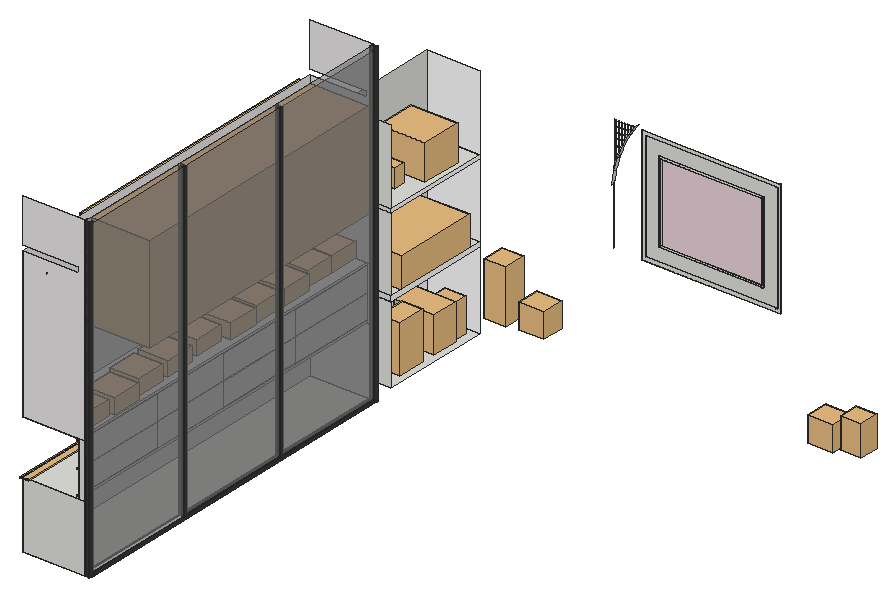
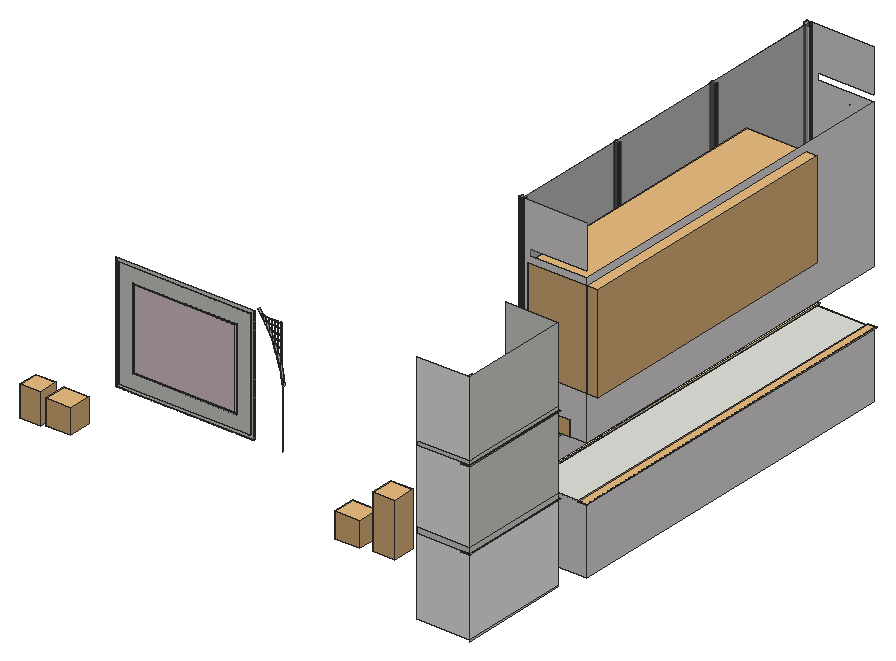
# SketchUp Ruby script. Lengths in inches.
U = 1.inch
M = Sketchup.active_model
def pt(a) = Geom::Point3d.new(a.map { |v| v * U })
def face(e, loops, mat)
  f = e.add_face(loops[0].map { |a| pt(a) })
  loops[1..].each { |l| e.add_face(l.map { |a| pt(a) }).erase! }
  f.material = f.back_material = mat if mat
  f
end
# faces: each face lists its corners as indices into pts; further lists are holes
def faces(e, pts, list, mat = nil) = list.each { |f| face(e, (f[0].is_a?(Array) ? f : [f]).map { |l| l.map { |i| pts[i] } }, mat) }
# xy, xz, yz: faces in a plane at the given z, y or x. An outline is a flat list of corners, or four numbers for a rectangle; further outlines are holes
def ring(l) = l.size == 4 ? [[l[0], l[1]], [l[2], l[1]], [l[2], l[3]], [l[0], l[3]]] : l.each_slice(2).to_a
def flat(e, list, mat, &to3) = list.each { |f| face(e, (f[0].is_a?(Array) ? f : [f]).map { |l| ring(l).map { |u, v| to3.(u, v) } }, mat) }
def xy(e, z, list, mat = nil) = flat(e, list, mat) { |x, y| [x, y, z] }
def xz(e, y, list, mat = nil) = flat(e, list, mat) { |x, z| [x, y, z] }
def yz(e, x, list, mat = nil) = flat(e, list, mat) { |y, z| [x, y, z] }
def lines(e, pts, list) = list.each { |a, b| e.add_line(pt(pts[a]), pt(pts[b])) }
# prism: a flat outline (further loops are holes) pulled along v
def prism(e, loops, v, mat = nil)
  f = face(e, loops, mat); d = Geom::Vector3d.new(v.map { |x| x * U })
  f.pushpull(f.normal.samedirection?(d) ? d.length : -d.length)
end
def box(e, o, s, mat = nil) = prism(e, [[o, [o[0] + s[0], o[1], o[2]], [o[0] + s[0], o[1] + s[1], o[2]], [o[0], o[1] + s[1], o[2]]]], [0, 0, s[2]], mat)
def at(x, y, z, deg = 0) = Geom::Transformation.translation(pt([x, y, z])) * Geom::Transformation.rotation(ORIGIN, Z_AXIS, deg.degrees)
def axes(o, x, y, z) = Geom::Transformation.new([*x, 0, *y, 0, *z, 0, *pt(o).to_a, 1])
def part(name) = M.definitions.add(name)
# library, detail: a bought-in or finely detailed component or shape, given as its bounding box
def library(name, o, s) = part(name).tap { |d| box(d.entities, o, s) }
def detail(e, o, s) = box(e.add_group.entities, o, s)
def put(e, d, t, mat = nil) = e.add_instance(d, t).tap { |i| i.material = mat if mat }
def group(e, t, mat = nil) = e.add_group.tap { |g| g.transformation = t; g.material = mat if mat }.entities
root = M.entities
M.materials.add("Generic").color = [234, 232, 232]
M.materials.add("Gold 10k").color = [251, 232, 180]
M.materials.add("[Color M00]").color = [255, 255, 255]
M.materials.add("[Color M02]").color = [237, 213, 220]
M.materials.add("[Color M07]").color = [58, 58, 58]
M.materials.add("[Translucent Glass Gray]").color = [128, 128, 128]
M.materials["[Translucent Glass Gray]"].alpha = 0.5
c1 = library("Interior Props 221 031",[-3.74,-3.52,-0.04],[7.48,7.03,11.78])
c2 = library("Interior Props 221 030",[-2.57,-3.63,-0.04],[5.13,7.27,11.89])
c3 = library("Interior Props 221 029",[-1.46,-2.15,0],[2.92,4.3,3.83])
c4 = library("Lamp Table 025",[-4.92,-4.92,-0.03],[22.02,19.61,21.68])
c5 = library("Potted Succulent 003",[-4.09,-3.62,0],[7.1,6.83,10.79])
c6 = library("Potted Basil 50-07",[-3.85,-3.53,0.03],[7.56,8,18.65])
c7 = library("Group\#7",[-0.5,-0.5,-0.1],[3,127.16,0.2])
c8 = library("Group\#1",[-0.5,-0.5,-0.1],[3,40,0.2])
c9 = library("Bowls and Vases 20-14",[-14.94,-8.87,0],[29.88,17.74,10.58])
c10 = library("Clothes 159 005",[-5.11,-5.34,0.03],[10.26,10.67,5.26])
c11 = library("Group\#4",[-0.5,-0.5,-0.1],[3,40,0.2])
c12 = library("Interior Props 160 011",[-3.43,-7.07,0],[14.06,16.26,12.45])
c13 = library("Perfume 101 004",[-2,-2,-0.02],[4,4,6.5])
c14 = library("Clothing 209 002",[69.11,63.18,62.21],[24.57,96.36,33.87])
xy(root,4.07,[[11.1875,11.43,33,137.59],[33,11.43,33.4375,12.43],[33.4375,11.43,34.4375,12.43],[34.4375,11.43,34.8125,12.43],[33,136.59,33.4375,137.59],
  [33.4375,136.59,34.4375,137.59],[34.4375,136.59,34.8125,137.59]])
xy(root,4.07,[[33,12.43,33.4375,136.59],[33.4375,12.43,34.4375,136.59],[34.4375,12.43,34.8125,136.59]],"[Color M07]")
xy(root,4.17,[[14.5,145.84,33,184.83]])
xy(root,5.07,[[33,12.43,34.4375,52.82],[33,52.82,34.4375,53.82],[34.4375,52.82,34.8125,53.82],[33,95.21,34.4375,96.21],[34.4375,95.21,34.8125,96.21]])
xy(root,5.07,[[34.4375,12.43,34.8125,52.82],[33,53.82,34.4375,95.21],[34.4375,53.82,34.8125,95.21],[33,96.21,34.4375,136.59],[34.4375,96.21,34.8125,136.59]],"[Color M07]")
xy(root,27.47,[[13.1875,11.43,31,137.59]])
xy(root,28.22,[[30.25,11.43,31,137.59]],"Gold 10k")
xy(root,28.62,[[30.25,11.43,31,45.36],[30.25,45.76,31,74.51],[30.25,74.91,31,106.25],[30.25,106.65,31,137.59]],"Gold 10k")
xy(root,31.38,[[16.5,145.84,33,184.83]])
xy(root,33.15,[[14.5,145.84,33,184.83]])
xy(root,36.62,[[30.25,11.43,31,45.36],[30.25,45.76,31,74.51],[30.25,74.91,31,106.25],[30.25,106.65,31,137.59]],"Gold 10k")
xy(root,37.02,[[30.25,11.43,31,45.36],[30.25,45.76,31,74.51],[30.25,74.91,31,106.25],[30.25,106.65,31,137.59]],"Gold 10k")
xy(root,44.04,[[86.13,189.625,86.13,189.8125,86.26,189.8125,86.26,189.875,86.82,189.875,86.82,189.8125,87.42,189.8125,87.42,189.875,87.99,189.875,87.99,189.8125,88.58,189.8125,88.58,189.875,89.15,189.875,89.15,189.8125,89.75,189.8125,89.75,189.875,90.3125,189.875,90.3125,189.8125,90.91,189.8125,90.91,189.875,91.48,189.875,91.48,189.8125,92.08,189.8125,92.08,189.875,92.64,189.875,92.64,189.8125,93.24,189.8125,93.24,189.875,93.8,189.875,93.8,189.8125,94.4,189.8125,94.4,189.875,94.97,189.875,94.97,189.8125,95.57,189.8125,95.57,189.875,96.13,189.875,96.13,189.8125,96.73,189.8125,96.73,189.875,97.29,189.875,97.29,189.8125,97.89,189.8125,97.89,189.875,98.46,189.875,98.46,189.8125,99.06,189.8125,99.06,189.875,99.62,189.875,99.62,189.8125,100.22,189.8125,100.22,189.875,100.79,189.875,100.79,189.8125,101.38,189.8125,101.38,189.875,101.95,189.875,101.95,189.8125,102.55,189.8125,102.55,189.875,103.11,189.875,103.11,189.8125,103.71,189.8125,103.71,189.875,104.28,189.875,104.28,189.8125,104.875,189.8125,104.875,189.875,105.28,189.875,105.28,189.8125,105.875,189.8125,105.875,189.875,106.28,189.875,106.28,189.8125,106.875,189.8125,106.875,189.875,107.28,189.875,107.28,189.8125,107.875,189.8125,107.875,189.875,108.28,189.875,108.28,189.8125,108.875,189.8125,108.875,189.875,109.28,189.875,109.28,189.8125,109.875,189.8125,109.875,189.875,110.28,189.875,110.28,189.8125,110.875,189.8125,110.875,189.875,111.28,189.875,111.28,189.8125,111.875,189.8125,111.875,189.875,112.28,189.875,112.28,189.8125,112.875,189.8125,112.875,189.875,113.28,189.875,113.28,189.8125,113.875,189.8125,113.875,189.875,114.28,189.875,114.28,189.8125,114.875,189.8125,114.875,189.875,115.28,189.875,115.28,189.8125,115.875,189.8125,115.875,189.875,116.28,189.875,116.28,189.8125,116.875,189.8125,116.875,189.875,117.28,189.875,117.28,189.8125,117.875,189.8125,117.875,189.875,118.28,189.875,118.28,189.8125,118.875,189.8125,118.875,189.875,119.28,189.875,119.28,189.8125,119.875,189.8125,119.875,189.875,120.28,189.875,120.28,189.8125,120.875,189.8125,120.875,189.875,121.28,189.875,121.28,189.8125,121.875,189.8125,121.875,189.875,122.28,189.875,122.28,189.8125,122.875,189.8125,122.875,189.875,123.28,189.875,123.28,189.8125,123.875,189.8125,123.875,189.875,124.28,189.875,124.28,189.75,124.875,189.75,124.875,189.875,125.28,189.875,125.28,189.75,125.875,189.75,125.875,189.875,126.28,189.875,126.28,189.75,126.875,189.75,126.875,189.875,127.28,189.875,127.28,189.75,127.875,189.75,127.875,189.875,128.28,189.875,128.28,189.75,128.875,189.75,128.875,189.875,129.28,189.875,129.28,189.75,129.875,189.75,129.875,189.875,130.28,189.875,130.28,189.75,130.875,189.75,130.875,189.875,131.28,189.875,131.28,189.75,131.875,189.75,131.875,189.875,132.28,189.875,132.28,189.75,132.875,189.75,132.875,189.875,133.28,189.875,133.28,189.75,133.875,189.75,133.875,189.875,134.28,189.875,134.28,189.625],[134.28,189.625,134.75,189.875],[131.28,189.75,131.75,189.875],[131.75,189.75,131.875,189.875],[132.28,189.75,132.75,189.875],
  [132.75,189.75,132.875,189.875],[133.28,189.75,133.75,189.875],[133.75,189.75,133.875,189.875],[86.13,189.8125,86.14,189.875],[86.14,189.8125,86.26,189.875]])
xy(root,45.1875,[[87.28,189.625,133.61,189.875]])
xy(root,45.36,[[30.25,106.65,31,137.59]],"Gold 10k")
xy(root,45.42,[[30.25,45.76,31,45.77]])
xy(root,45.42,[[30.25,11.43,31,45.36],[30.25,45.77,31,74.51],[30.25,74.91,31,106.25]],"Gold 10k")
xy(root,45.82,[[30.25,11.43,31,137.59]],"Gold 10k")
xy(root,46.57,[[11.1875,11.43,31,137.59]],"Generic")
xy(root,50.04,[[92.125,189.625,128.76,189.875]])
xy(root,50.62,[[92.71,189.625,128.18,189.875]])
xy(root,59.13,[[16.5,145.84,33,184.83]])
xy(root,60.4,[[14.5,145.84,33,184.83]])
xy(root,78.09,[[92.71,189.625,128.18,189.875]])
xy(root,78.67,[[92.125,189.625,128.76,189.875]])
xy(root,83.52,[[87.28,189.625,133.61,189.875]])
xz(root,11.43,[[11.1875,4.07,33,27.47],[31,27.47,31,28.22,30.25,28.22,30.25,28.62,31,28.62,31,36.62,30.25,36.62,30.25,37.02,31,37.02,31,45.42,30.25,45.42,30.25,45.82,31,45.82,31,46.57,33,46.57,33,27.47]])
xz(root,11.43,[[[11.1875,46.57,11.1875,98.59,31,98.59,31,100.64,11.1875,100.64,11.1875,115.93,33,115.93,33,46.57],[19.57,94.12,19.68,94.13,19.77,94.17,19.86,94.23,19.92,94.32,19.96,94.41,19.97,94.52,19.96,94.62,19.92,94.72,19.86,94.8,19.77,94.86,19.68,94.9,19.57,94.92,19.47,94.9,19.37,94.86,19.29,94.8,19.23,94.72,19.1875,94.62,19.17,94.52,19.1875,94.41,19.23,94.32,19.29,94.23,19.37,94.17,19.47,94.13]]],"Generic")
xz(root,11.43,[[33,4.07,33.4375,115.93],[33.4375,4.07,34.4375,115.93],[34.4375,4.07,34.8125,115.93]],"[Color M07]")
xz(root,12.43,[[33,4.07,34.4375,5.07],[34.4375,4.07,34.8125,5.07],[33,5.07,34.4375,114.93]])
xz(root,12.43,[[34.4375,5.07,34.8125,114.93]],"[Color M07]")
xz(root,45.36,[[30.25,28.62,31,36.62],[30.25,37.02,31,45.42]],"Gold 10k")
xz(root,45.76,[[30.25,28.62,31,36.62],[30.25,37.02,31,45.42]],"Gold 10k")
xz(root,52.82,[[33,5.07,34.4375,114.93],[34.4375,5.07,34.8125,114.93]],"[Color M07]")
xz(root,53.82,[[33,5.07,34.4375,114.93],[34.4375,5.07,34.8125,114.93]],"[Color M07]")
xz(root,74.51,[[30.25,28.62,31,36.62],[30.25,37.02,31,45.42]],"Gold 10k")
xz(root,74.91,[[30.25,28.62,31,36.62],[30.25,37.02,31,45.42]],"Gold 10k")
xz(root,95.21,[[33,5.07,34.4375,114.93],[34.4375,5.07,34.8125,114.93]],"[Color M07]")
xz(root,96.21,[[33,5.07,34.4375,114.93],[34.4375,5.07,34.8125,114.93]],"[Color M07]")
xz(root,106.25,[[30.25,28.62,31,36.62],[30.25,37.02,31,45.42]],"Gold 10k")
xz(root,106.65,[[30.25,28.62,31,36.62],[30.25,37.02,31,45.36]],"Gold 10k")
xz(root,136.59,[[33,4.07,34.4375,5.07],[34.4375,4.07,34.8125,5.07]])
xz(root,136.59,[[33,5.07,34.4375,114.93],[34.4375,5.07,34.8125,114.93]],"[Color M07]")
xz(root,137.59,[[11.1875,4.07,33,27.47],[31,27.47,33,27.47,33,46.57,31,46.57,31,45.82,30.25,45.82,30.25,45.36,31,45.36,31,37.02,30.25,37.02,30.25,36.62,31,36.62,31,28.62,30.25,28.62,30.25,28.22,31,28.22],[[11.1875,46.57,33,46.57,33,115.93,11.1875,115.93,11.1875,100.64,31,100.64,31,98.59,11.1875,98.59],[19.57,94.12,19.47,94.13,19.37,94.17,19.29,94.23,19.23,94.32,19.1875,94.41,19.17,94.52,19.1875,94.62,19.23,94.72,19.29,94.8,19.37,94.86,19.47,94.9,19.57,94.92,19.68,94.9,19.77,94.86,19.86,94.8,19.92,94.72,19.96,94.62,19.97,94.52,19.96,94.41,19.92,94.32,19.86,94.23,19.77,94.17,19.68,94.13]]],"Generic")
xz(root,137.59,[[33,4.07,33.4375,115.93],[33.4375,4.07,34.4375,115.93],[34.4375,4.07,34.8125,115.93]],"[Color M07]")
xz(root,145.84,[[14.5,4.17,33,31.38],[14.5,31.38,33,33.15],[14.5,33.15,33,59.13],[14.5,59.13,33,60.4],[14.5,60.4,33,86.88]])
xz(root,184.83,[[14.5,31.38,33,33.15],[14.5,59.13,33,60.4]])
xz(root,184.83,[[14.5,4.17,33,31.38],[14.5,33.15,33,59.13],[14.5,60.4,33,86.88]],"[Color M00]")
xz(root,189.625,[[[86.13,44.04,134.75,84.67],[87.28,45.1875,133.61,83.52]],[[92.125,50.04,128.76,78.67],[92.71,50.62,128.18,78.09]]])
xz(root,189.875,[[76,44.04,76.0625,44.04,76.0625,64.2,76.6,67.64,76.6,71.82,76,69.625],[86.13,44.04,86.26,84.67],[134.28,44.04,134.75,84.67],[[87.28,45.1875,133.61,83.52],[92.125,50.04,128.76,78.67]],[77,69.625,77.6,71.82,77.6,74.82,77.03,73.375,77,73.29],
  [78,73.29,78.03,73.375,78.6,74.82,78.6,77.35,78,75.84],[79,75.84,79.6,77.35,79.6,79.33,79,78.2],[80,78.2,80.6,79.33,80.6,81.21,80,80.08],[81,80.08,81.6,81.21,81.6,83.06,81,82.1875],[82.17,82.1875,82.77,83.06,82.77,84.67,82.7,84.67,82.17,83.89],
  [83.33,83.89,83.86,84.67,83.33,84.67]])
xz(root,189.875,[[92.71,50.62,128.18,78.09]],"[Color M02]")
yz(root,11.1875,[[11.43,4.07,137.59,27.47],[11.43,46.57,137.59,98.59]],"Generic")
yz(root,14.5,[[145.84,3.63,184.83,4.17],[145.84,31.38,184.83,33.15],[145.84,33.15,184.83,59.13],[145.84,59.13,184.83,60.4],[145.84,60.4,184.83,86.88]])
yz(root,14.5,[[145.84,4.17,184.83,31.38]],"[Color M00]")
yz(root,30.25,[[[11.43,28.22,137.59,28.22,137.59,28.62,106.65,28.62,106.65,36.62,137.59,36.62,137.59,37.02,106.65,37.02,106.65,45.36,137.59,45.36,137.59,45.82,11.43,45.82,11.43,45.42,45.36,45.42,45.36,37.02,11.43,37.02,11.43,36.62,45.36,36.62,45.36,28.62,11.43,28.62],[74.91,37.02,106.25,45.42],[74.91,28.62,106.25,36.62],[45.76,37.02,74.51,45.42],[45.76,28.62,74.51,36.62]]],"Gold 10k")
yz(root,31,[[11.43,27.47,137.59,28.22],[11.43,28.62,45.36,36.62],[45.76,28.62,74.51,36.62],[74.91,28.62,106.25,36.62],[106.65,28.62,137.59,36.62],
  [11.43,37.02,45.36,45.42],[45.76,37.02,74.51,45.42],[74.91,37.02,106.25,45.42],[106.65,37.02,137.59,45.36],[11.43,45.82,137.59,46.57]],"Generic")
yz(root,33,[[145.84,31.38,184.83,33.15],[145.84,59.13,184.83,60.4]],"[Color M00]")
yz(root,33,[[11.43,4.07,12.43,115.93],[12.43,4.07,136.59,5.07],[136.59,4.07,137.59,115.93],[52.82,5.07,53.82,114.93],[95.21,5.07,96.21,114.93]],"[Color M07]")
yz(root,33.4375,[[11.43,4.07,137.59,115.93]],"[Translucent Glass Gray]")
yz(root,34.4375,[[11.43,4.07,12.43,115.93],[12.43,4.07,136.59,5.07],[136.59,4.07,137.59,115.93],[52.82,5.07,53.82,114.93],[95.21,5.07,96.21,114.93]])
yz(root,34.4375,[[12.43,5.07,52.82,114.93],[53.82,5.07,95.21,114.93],[96.21,5.07,136.59,114.93]],"[Translucent Glass Gray]")
yz(root,34.8125,[[11.43,4.07,12.43,115.93],[12.43,4.07,136.59,5.07],[136.59,4.07,137.59,115.93],[52.82,5.07,53.82,114.93],[95.21,5.07,96.21,114.93]],"[Color M07]")
yz(root,76.0625,[[189.8125,44.04,189.875,64.2]])
yz(root,86.13,[[189.625,44.04,189.8125,84.67],[189.8125,44.04,189.875,84.67]])
yz(root,87.28,[[189.625,45.1875,189.875,83.52]])
yz(root,92.125,[[189.625,50.04,189.875,78.67]])
yz(root,92.71,[[189.625,50.62,189.875,78.09]])
yz(root,128.18,[[189.625,50.62,189.875,78.09]])
yz(root,128.76,[[189.625,50.04,189.875,78.67]])
yz(root,133.61,[[189.625,45.1875,189.875,83.52]])
yz(root,134.75,[[189.625,44.04,189.875,84.67]])
p = [[76.79,189,68.84],[76.0625,189,64.2],[76.0625,189.8125,64.2],[76.6,189.8125,67.64],[76.6,189.875,67.64],[76.79,189.875,68.84],
  [76.0625,189.875,64.2],[78.03,189,73.375],[77,189.875,69.625],[77,189.8125,69.625],[77.6,189.8125,71.82],[77.6,189.875,71.82],
  [78,189.875,73.29],[78,189.8125,73.29],[78.03,189.8125,73.375],[78.03,189.875,73.375],[79.76,189,77.74],[78.6,189.8125,74.82],
  [78.6,189.875,74.82],[79,189.875,75.84],[79,189.8125,75.84],[79.6,189.8125,77.35],[79.6,189.875,77.35],[79.76,189.875,77.74],
  [81.96,189,81.89],[80,189.875,78.2],[80,189.8125,78.2],[80.6,189.8125,79.33],[80.6,189.875,79.33],[81,189.875,80.08],
  [81,189.8125,80.08],[81.6,189.8125,81.21],[81.6,189.875,81.21],[81.96,189.875,81.89],[84.62,189,85.77],[82.17,189.875,82.1875],
  [82.17,189.8125,82.1875],[82.77,189.8125,83.06],[82.77,189.875,83.06],[83.33,189.875,83.89],[83.33,189.8125,83.89],[83.86,189.8125,84.67],
  [83.86,189.875,84.67],[84.28,189.875,85.28],[84.28,189.8125,85.28],[84.62,189.8125,85.77],[31,74.51,45.42],[31,74.53,45.42],
  [82.17,189.875,83.89],[82.17,189.875,84.67],[81.6,189.875,84.67],[81.6,189.875,83.06],[81,189.875,83.89],[81,189.875,84.67],
  [81.53,189.875,84.67],[81,189.875,82.1875],[80.53,189.875,84.67],[80,189.875,83.89],[80,189.875,82.1875],[80.6,189.875,83.06],
  [80.6,189.875,81.21],[80,189.875,80.08],[80.6,189.875,84.67],[80,189.875,84.67],[79,189.875,83.89],[79,189.875,84.67],
  [79.6,189.875,81.21],[79.6,189.875,79.33],[79.6,189.875,84.67],[79.6,189.875,83.06],[79.53,189.875,84.67],[79,189.875,82.1875],
  [79,189.875,78.2],[79,189.875,80.08],[78.6,189.875,84.67],[78.6,189.875,83.06],[78,189.875,83.89],[78,189.875,84.67],
  [78.6,189.875,81.21],[78.6,189.875,79.33],[78.53,189.875,84.67],[78,189.875,82.1875],[78,189.875,80.08],[78,189.875,78.2],
  [78,189.875,75.84],[78.6,189.875,77.35],[77.53,189.875,84.67],[77,189.875,83.89],[77,189.875,80.08],[77,189.875,82.1875],
  [77.6,189.875,77.35],[77,189.875,75.84],[77,189.875,84.67],[77,189.875,73.29],[77.6,189.875,81.21],[77.6,189.875,79.33],
  [77.6,189.875,84.67],[77.6,189.875,83.06],[77,189.875,78.2],[77.6,189.875,74.82],[76.6,189.875,79.33],[76.6,189.875,77.35],
  [76.6,189.875,74.82],[76,189.875,75.84],[76,189.875,78.2],[76.6,189.875,83.06],[76.6,189.875,81.21],[76.03,189.875,73.375],
  [76,189.875,73.29],[76.6,189.875,71.82],[76,189.875,80.08],[76.53,189.875,84.67],[76,189.875,83.89],[76.6,189.875,84.67],
  [76,189.875,82.1875],[76,189.875,84.67],[76,189.875,69.625]]
faces(root,p,[[0,1,2,3,4,5],[6,4,3,2],[7,0,5,8,9,10,11,12,13,14],[8,11,10,9],[12,15,14,13],[16,7,14,17,18,19,20,21,22,23],[15,18,17,14],[19,22,21,20],
  [24,16,23,25,26,27,28,29,30,31,32,33],[25,28,27,26],[29,32,31,30],[34,24,33,35,36,37,38,39,40,41,42,43,44,45],[35,38,37,36],[39,42,41,40]])
lines(root,p,[[46,47],[48,49],[50,51],[52,53],[54,52],[55,52],[56,57],[58,57],[59,58],[59,60],[61,58],[62,59],
  [57,63],[64,65],[66,67],[68,69],[70,64],[71,64],[69,71],[72,73],[69,66],[73,71],[66,73],[74,75],
  [76,77],[78,79],[80,76],[81,76],[82,81],[75,81],[79,83],[84,83],[75,78],[79,85],[78,82],[83,82],
  [86,87],[88,89],[90,91],[89,87],[87,92],[93,91],[94,95],[96,97],[97,89],[95,98],[91,98],[95,90],
  [94,88],[98,88],[90,99],[97,94],[100,101],[101,102],[103,104],[105,106],[102,107],[107,108],[102,109],[104,110],
  [106,110],[111,112],[113,105],[105,114],[114,112],[108,103],[110,114],[101,103],[112,115],[106,100],[100,104],[116,108]])
put(root,c1,at(26.23,179,4.17))
put(root,c2,axes([26.91,157.73,4.18],[1.39,0,0],[0,1.39,0],[0,0,1.39]))
put(root,c3,axes([23.53,172.35,4.16],[0,3.29,0],[-3.29,0,0],[0,0,3.29]))
put(root,c4,axes([56.93,176.47,17.7],[0.4,0,0],[0,0.4,0],[0,0,0.4]))
put(root,c4,axes([158.24,176.47,17.7],[0.4,0,0],[0,0.4,0],[0,0,0.4]))
put(root,c5,at(170.09,180.48,17.72))
put(root,c6,at(47.38,176.97,17.6875))
put(root,c7,at(11.1875,11.43,27.47))
put(root,c8,at(14.5,145.84,31.38))
put(root,c9,at(24.13,165.26,33.15,90))
put(root,c10,at(25.18,33.19,46.57))
put(root,c10,at(23.65,45.66,46.57))
put(root,c10,at(23.33,58.6,46.57))
put(root,c10,at(24.47,20.99,46.57))
put(root,c10,at(22.14,72.79,46.57))
put(root,c10,at(23.86,85.98,46.57))
put(root,c10,at(23.48,97.63,46.57))
put(root,c10,at(23.35,109.92,46.57))
put(root,c10,at(21.88,121.9,46.57))
put(root,c10,at(22,132.4,46.57))
put(root,c11,at(14.5,145.84,59.13))
put(root,c12,at(23.85,166.86,60.4,90))
put(root,c13,at(24.54,157.32,60.42))
put(root,c14,at(-61.8125,-21.94,0))
